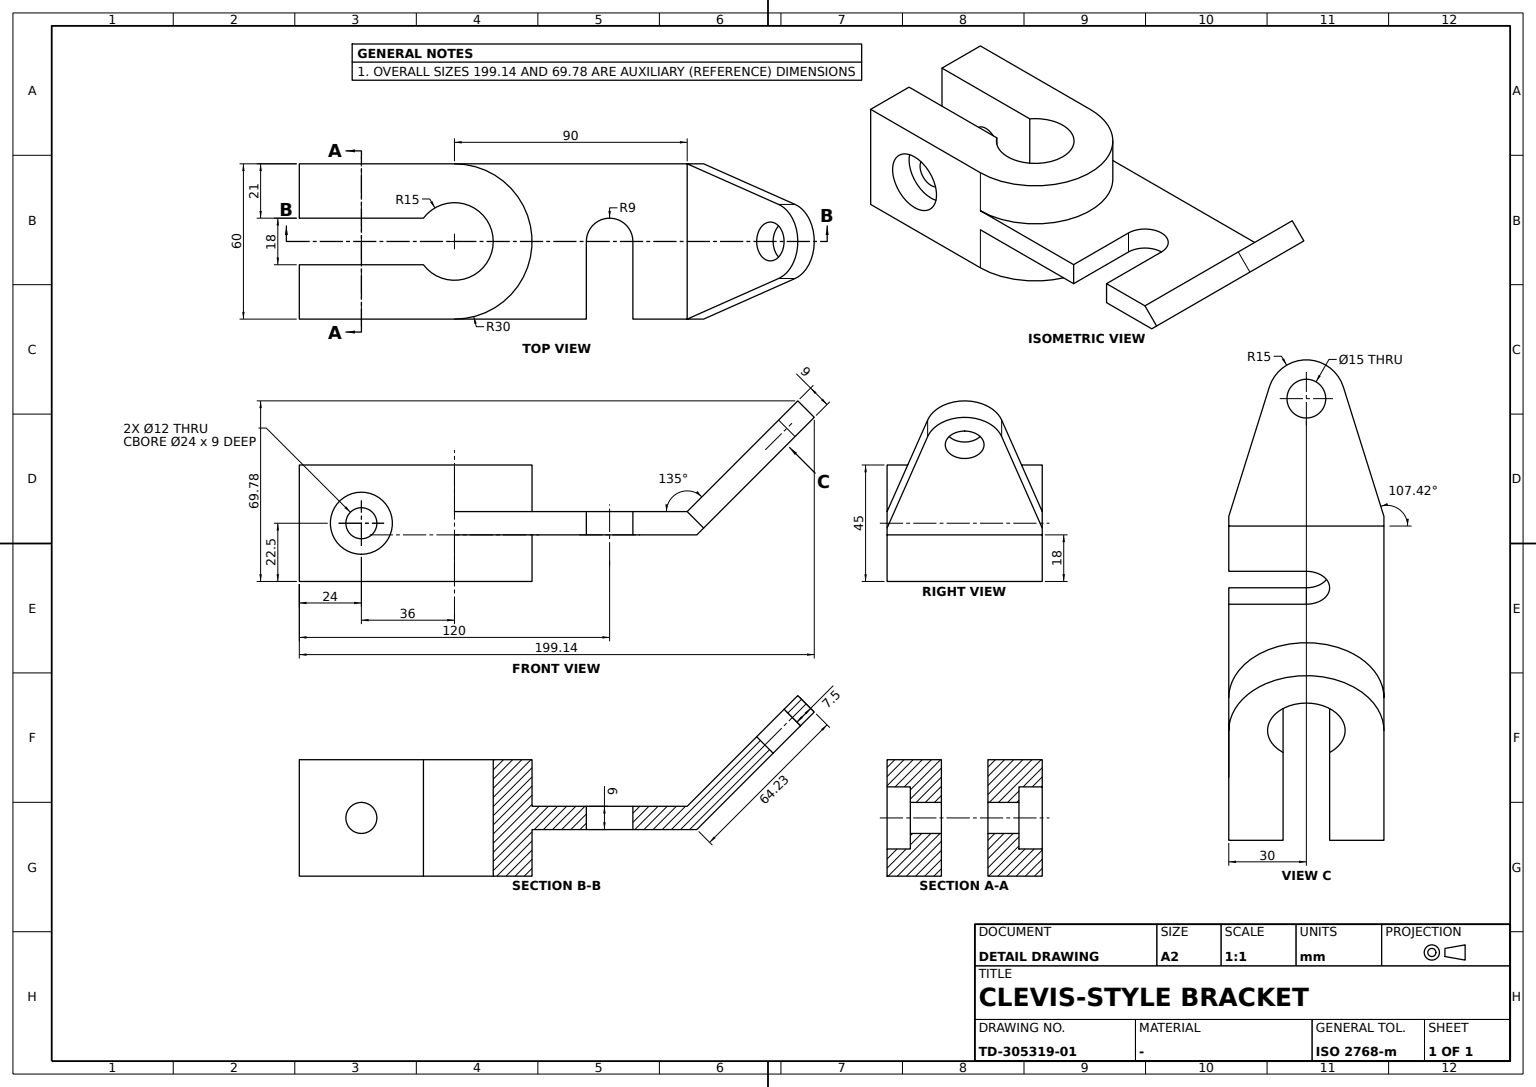
ISO-10303-21;
HEADER;
FILE_DESCRIPTION((''),'2;1');
FILE_NAME('','',(''),(''),'','','');
FILE_SCHEMA(('AUTOMOTIVE_DESIGN'));
ENDSEC;
DATA;
#1=APPLICATION_CONTEXT('');
#2=PRODUCT_CONTEXT('',#1,'mechanical');
#3=PRODUCT('','','',(#2));
#4=PRODUCT_DEFINITION_FORMATION('','',#3);
#5=PRODUCT_DEFINITION_CONTEXT('',#1,'design');
#6=PRODUCT_DEFINITION('','',#4,#5);
#7=PRODUCT_DEFINITION_SHAPE('','',#6);
#8=(LENGTH_UNIT()NAMED_UNIT(*)SI_UNIT(.MILLI.,.METRE.));
#9=(NAMED_UNIT(*)PLANE_ANGLE_UNIT()SI_UNIT($,.RADIAN.));
#10=(NAMED_UNIT(*)SI_UNIT($,.STERADIAN.)SOLID_ANGLE_UNIT());
#11=UNCERTAINTY_MEASURE_WITH_UNIT(LENGTH_MEASURE(0.005),#8,'distance_accuracy_value','');
#12=(GEOMETRIC_REPRESENTATION_CONTEXT(3)GLOBAL_UNCERTAINTY_ASSIGNED_CONTEXT((#11))GLOBAL_UNIT_ASSIGNED_CONTEXT((#8,#9,#10))REPRESENTATION_CONTEXT('',''));
#13=CARTESIAN_POINT('',(21.,-36.,6.));
#14=VERTEX_POINT('',#13);
#15=CARTESIAN_POINT('',(21.,-36.,0.));
#16=DIRECTION('',(-1.,0.,0.));
#17=DIRECTION('',(0.,0.,1.));
#18=AXIS2_PLACEMENT_3D('',#15,#16,#17);
#19=CIRCLE('',#18,6.);
#20=EDGE_CURVE('',#14,#14,#19,.T.);
#21=ORIENTED_EDGE('',*,*,#20,.T.);
#22=EDGE_LOOP('',(#21));
#23=FACE_BOUND('',#22,.T.);
#24=CARTESIAN_POINT('',(21.,-36.,12.));
#25=VERTEX_POINT('',#24);
#26=CIRCLE('',#18,12.);
#27=EDGE_CURVE('',#25,#25,#26,.T.);
#28=ORIENTED_EDGE('',*,*,#27,.F.);
#29=EDGE_LOOP('',(#28));
#30=FACE_BOUND('',#29,.T.);
#31=CARTESIAN_POINT('',(21.,-30.,0.));
#32=DIRECTION('',(0.,1.,0.));
#33=AXIS2_PLACEMENT_3D('',#31,#16,#32);
#34=PLANE('',#33);
#35=ADVANCED_FACE('',(#23,#30),#34,.F.);
#36=CARTESIAN_POINT('',(-30.,0.,22.5));
#37=VERTEX_POINT('',#36);
#38=CARTESIAN_POINT('',(-30.,-60.,22.5));
#39=VERTEX_POINT('',#38);
#40=DIRECTION('',(0.,-1.,0.));
#41=VECTOR('',#40,1000.);
#42=LINE('',#36,#41);
#43=EDGE_CURVE('',#37,#39,#42,.T.);
#44=ORIENTED_EDGE('',*,*,#43,.F.);
#45=CARTESIAN_POINT('',(-30.,0.,4.5));
#46=VERTEX_POINT('',#45);
#47=CARTESIAN_POINT('',(-30.,0.,0.));
#48=VECTOR('',#17,1000.);
#49=LINE('',#47,#48);
#50=EDGE_CURVE('',#46,#37,#49,.T.);
#51=ORIENTED_EDGE('',*,*,#50,.F.);
#52=CARTESIAN_POINT('',(-30.,90.,4.5));
#53=VERTEX_POINT('',#52);
#54=LINE('',#52,#41);
#55=EDGE_CURVE('',#53,#46,#54,.T.);
#56=ORIENTED_EDGE('',*,*,#55,.F.);
#57=CARTESIAN_POINT('',(-30.,96.363961,-1.863961));
#58=VERTEX_POINT('',#57);
#59=CARTESIAN_POINT('',(-30.,47.25,47.25));
#60=DIRECTION('',(0.,0.707106781,-0.707106781));
#61=VECTOR('',#60,1000.);
#62=LINE('',#59,#61);
#63=EDGE_CURVE('',#53,#58,#62,.T.);
#64=ORIENTED_EDGE('',*,*,#63,.T.);
#65=CARTESIAN_POINT('',(-30.,93.727922,-4.5));
#66=VERTEX_POINT('',#65);
#67=DIRECTION('',(0.,0.707106781,0.707106781));
#68=VECTOR('',#67,1000.);
#69=LINE('',#65,#68);
#70=EDGE_CURVE('',#66,#58,#69,.T.);
#71=ORIENTED_EDGE('',*,*,#70,.F.);
#72=CARTESIAN_POINT('',(-30.,0.,-4.5));
#73=VERTEX_POINT('',#72);
#74=VECTOR('',#32,1000.);
#75=LINE('',#72,#74);
#76=EDGE_CURVE('',#73,#66,#75,.T.);
#77=ORIENTED_EDGE('',*,*,#76,.F.);
#78=CARTESIAN_POINT('',(-30.,0.,-22.5));
#79=VERTEX_POINT('',#78);
#80=EDGE_CURVE('',#79,#73,#49,.T.);
#81=ORIENTED_EDGE('',*,*,#80,.F.);
#82=CARTESIAN_POINT('',(-30.,-60.,-22.5));
#83=VERTEX_POINT('',#82);
#84=LINE('',#78,#41);
#85=EDGE_CURVE('',#79,#83,#84,.T.);
#86=ORIENTED_EDGE('',*,*,#85,.T.);
#87=CARTESIAN_POINT('',(-30.,-60.,0.));
#88=LINE('',#87,#48);
#89=EDGE_CURVE('',#83,#39,#88,.T.);
#90=ORIENTED_EDGE('',*,*,#89,.T.);
#91=EDGE_LOOP('',(#44,#51,#56,#64,#71,#77,#81,#86,#90));
#92=FACE_BOUND('',#91,.T.);
#93=CARTESIAN_POINT('',(-30.,-36.,12.));
#94=VERTEX_POINT('',#93);
#95=CARTESIAN_POINT('',(-30.,-36.,0.));
#96=AXIS2_PLACEMENT_3D('',#95,#16,#17);
#97=CIRCLE('',#96,12.);
#98=EDGE_CURVE('',#94,#94,#97,.T.);
#99=ORIENTED_EDGE('',*,*,#98,.F.);
#100=EDGE_LOOP('',(#99));
#101=FACE_BOUND('',#100,.T.);
#102=AXIS2_PLACEMENT_3D('',#47,#16,#40);
#103=PLANE('',#102);
#104=ADVANCED_FACE('',(#92,#101),#103,.T.);
#105=CARTESIAN_POINT('',(0.,69.,4.5));
#106=VERTEX_POINT('',#105);
#107=CARTESIAN_POINT('',(0.,69.,-4.5));
#108=VERTEX_POINT('',#107);
#109=CARTESIAN_POINT('',(0.,69.,-9.66));
#110=LINE('',#109,#48);
#111=EDGE_CURVE('',#106,#108,#110,.F.);
#112=ORIENTED_EDGE('',*,*,#111,.F.);
#113=CARTESIAN_POINT('',(0.,51.,4.5));
#114=VERTEX_POINT('',#113);
#115=CARTESIAN_POINT('',(0.,60.,4.5));
#116=DIRECTION('',(1.,0.,0.));
#117=AXIS2_PLACEMENT_3D('',#115,#17,#116);
#118=CIRCLE('',#117,9.);
#119=EDGE_CURVE('',#106,#114,#118,.T.);
#120=ORIENTED_EDGE('',*,*,#119,.T.);
#121=CARTESIAN_POINT('',(0.,51.,-4.5));
#122=VERTEX_POINT('',#121);
#123=CARTESIAN_POINT('',(0.,51.,-9.66));
#124=LINE('',#123,#48);
#125=EDGE_CURVE('',#114,#122,#124,.F.);
#126=ORIENTED_EDGE('',*,*,#125,.T.);
#127=CARTESIAN_POINT('',(0.,60.,-4.5));
#128=DIRECTION('',(0.,0.,-1.));
#129=AXIS2_PLACEMENT_3D('',#127,#128,#16);
#130=CIRCLE('',#129,9.);
#131=EDGE_CURVE('',#122,#108,#130,.T.);
#132=ORIENTED_EDGE('',*,*,#131,.T.);
#133=EDGE_LOOP('',(#112,#120,#126,#132));
#134=FACE_BOUND('',#133,.T.);
#135=CARTESIAN_POINT('',(0.,60.,-9.66));
#136=AXIS2_PLACEMENT_3D('',#135,#17,#116);
#137=CYLINDRICAL_SURFACE('',#136,9.);
#138=ADVANCED_FACE('',(#134),#137,.F.);
#139=CARTESIAN_POINT('',(9.,-36.,-6.));
#140=VERTEX_POINT('',#139);
#141=CARTESIAN_POINT('',(9.,-36.,0.));
#142=AXIS2_PLACEMENT_3D('',#141,#116,#128);
#143=CIRCLE('',#142,6.);
#144=EDGE_CURVE('',#140,#140,#143,.T.);
#145=ORIENTED_EDGE('',*,*,#144,.F.);
#146=EDGE_LOOP('',(#145));
#147=FACE_BOUND('',#146,.T.);
#148=ORIENTED_EDGE('',*,*,#20,.F.);
#149=EDGE_LOOP('',(#148));
#150=FACE_BOUND('',#149,.T.);
#151=CARTESIAN_POINT('',(-29.9,-36.,0.));
#152=AXIS2_PLACEMENT_3D('',#151,#116,#32);
#153=CYLINDRICAL_SURFACE('',#152,6.);
#154=ADVANCED_FACE('',(#147,#150),#153,.F.);
#155=CARTESIAN_POINT('',(30.,0.,4.5));
#156=VERTEX_POINT('',#155);
#157=CARTESIAN_POINT('',(30.,0.,22.5));
#158=VERTEX_POINT('',#157);
#159=CARTESIAN_POINT('',(30.,0.,0.));
#160=LINE('',#159,#48);
#161=EDGE_CURVE('',#156,#158,#160,.T.);
#162=ORIENTED_EDGE('',*,*,#161,.F.);
#163=CARTESIAN_POINT('',(0.,0.,4.5));
#164=AXIS2_PLACEMENT_3D('',#163,#17,#116);
#165=CIRCLE('',#164,30.);
#166=EDGE_CURVE('',#156,#46,#165,.T.);
#167=ORIENTED_EDGE('',*,*,#166,.T.);
#168=ORIENTED_EDGE('',*,*,#50,.T.);
#169=CARTESIAN_POINT('',(0.,0.,22.5));
#170=AXIS2_PLACEMENT_3D('',#169,#17,#116);
#171=CIRCLE('',#170,30.);
#172=EDGE_CURVE('',#158,#37,#171,.T.);
#173=ORIENTED_EDGE('',*,*,#172,.F.);
#174=EDGE_LOOP('',(#162,#167,#168,#173));
#175=FACE_BOUND('',#174,.T.);
#176=CARTESIAN_POINT('',(0.,0.,0.));
#177=AXIS2_PLACEMENT_3D('',#176,#17,#32);
#178=CYLINDRICAL_SURFACE('',#177,30.);
#179=ADVANCED_FACE('',(#175),#178,.T.);
#180=ORIENTED_EDGE('',*,*,#144,.T.);
#181=EDGE_LOOP('',(#180));
#182=FACE_BOUND('',#181,.T.);
#183=CARTESIAN_POINT('',(9.,-12.,-22.5));
#184=VERTEX_POINT('',#183);
#185=CARTESIAN_POINT('',(9.,-60.,-22.5));
#186=VERTEX_POINT('',#185);
#187=LINE('',#183,#41);
#188=EDGE_CURVE('',#184,#186,#187,.T.);
#189=ORIENTED_EDGE('',*,*,#188,.T.);
#190=CARTESIAN_POINT('',(9.,-60.,22.5));
#191=VERTEX_POINT('',#190);
#192=CARTESIAN_POINT('',(9.,-60.,0.));
#193=VECTOR('',#128,1000.);
#194=LINE('',#192,#193);
#195=EDGE_CURVE('',#191,#186,#194,.T.);
#196=ORIENTED_EDGE('',*,*,#195,.F.);
#197=CARTESIAN_POINT('',(9.,-12.,22.5));
#198=VERTEX_POINT('',#197);
#199=LINE('',#197,#41);
#200=EDGE_CURVE('',#198,#191,#199,.T.);
#201=ORIENTED_EDGE('',*,*,#200,.F.);
#202=LINE('',#197,#48);
#203=EDGE_CURVE('',#198,#184,#202,.F.);
#204=ORIENTED_EDGE('',*,*,#203,.T.);
#205=EDGE_LOOP('',(#189,#196,#201,#204));
#206=FACE_BOUND('',#205,.T.);
#207=CARTESIAN_POINT('',(9.,-12.,0.));
#208=AXIS2_PLACEMENT_3D('',#207,#116,#40);
#209=PLANE('',#208);
#210=ADVANCED_FACE('',(#182,#206),#209,.F.);
#211=CARTESIAN_POINT('',(30.,93.727922,-4.5));
#212=VERTEX_POINT('',#211);
#213=CARTESIAN_POINT('',(30.,96.363961,-1.863961));
#214=VERTEX_POINT('',#213);
#215=CARTESIAN_POINT('',(30.,19.113961,-79.113961));
#216=LINE('',#215,#68);
#217=EDGE_CURVE('',#212,#214,#216,.T.);
#218=ORIENTED_EDGE('',*,*,#217,.T.);
#219=CARTESIAN_POINT('',(30.,90.,4.5));
#220=VERTEX_POINT('',#219);
#221=LINE('',#219,#61);
#222=EDGE_CURVE('',#220,#214,#221,.T.);
#223=ORIENTED_EDGE('',*,*,#222,.F.);
#224=CARTESIAN_POINT('',(30.,69.,4.5));
#225=VERTEX_POINT('',#224);
#226=CARTESIAN_POINT('',(30.,-60.,4.5));
#227=LINE('',#226,#41);
#228=EDGE_CURVE('',#220,#225,#227,.T.);
#229=ORIENTED_EDGE('',*,*,#228,.T.);
#230=CARTESIAN_POINT('',(30.,69.,-4.5));
#231=VERTEX_POINT('',#230);
#232=LINE('',#224,#193);
#233=EDGE_CURVE('',#225,#231,#232,.T.);
#234=ORIENTED_EDGE('',*,*,#233,.T.);
#235=CARTESIAN_POINT('',(30.,-60.,-4.5));
#236=LINE('',#235,#74);
#237=EDGE_CURVE('',#231,#212,#236,.T.);
#238=ORIENTED_EDGE('',*,*,#237,.T.);
#239=EDGE_LOOP('',(#218,#223,#229,#234,#238));
#240=FACE_BOUND('',#239,.T.);
#241=CARTESIAN_POINT('',(30.,-60.,0.));
#242=AXIS2_PLACEMENT_3D('',#241,#116,#32);
#243=PLANE('',#242);
#244=ADVANCED_FACE('',(#240),#243,.T.);
#245=CARTESIAN_POINT('',(30.,51.,4.5));
#246=VERTEX_POINT('',#245);
#247=CARTESIAN_POINT('',(30.,51.,-4.5));
#248=VERTEX_POINT('',#247);
#249=CARTESIAN_POINT('',(30.,51.,0.));
#250=LINE('',#249,#193);
#251=EDGE_CURVE('',#246,#248,#250,.T.);
#252=ORIENTED_EDGE('',*,*,#251,.T.);
#253=VECTOR('',#16,1000.);
#254=LINE('',#121,#253);
#255=EDGE_CURVE('',#248,#122,#254,.T.);
#256=ORIENTED_EDGE('',*,*,#255,.T.);
#257=ORIENTED_EDGE('',*,*,#125,.F.);
#258=LINE('',#245,#253);
#259=EDGE_CURVE('',#246,#114,#258,.T.);
#260=ORIENTED_EDGE('',*,*,#259,.F.);
#261=EDGE_LOOP('',(#252,#256,#257,#260));
#262=FACE_BOUND('',#261,.T.);
#263=AXIS2_PLACEMENT_3D('',#245,#40,#16);
#264=PLANE('',#263);
#265=ADVANCED_FACE('',(#262),#264,.F.);
#266=CARTESIAN_POINT('',(-9.,-60.,22.5));
#267=VERTEX_POINT('',#266);
#268=CARTESIAN_POINT('',(-9.,-60.,-22.5));
#269=VERTEX_POINT('',#268);
#270=CARTESIAN_POINT('',(-9.,-60.,0.));
#271=LINE('',#270,#193);
#272=EDGE_CURVE('',#267,#269,#271,.T.);
#273=ORIENTED_EDGE('',*,*,#272,.T.);
#274=CARTESIAN_POINT('',(-9.,-12.,-22.5));
#275=VERTEX_POINT('',#274);
#276=LINE('',#268,#74);
#277=EDGE_CURVE('',#269,#275,#276,.T.);
#278=ORIENTED_EDGE('',*,*,#277,.T.);
#279=CARTESIAN_POINT('',(-9.,-12.,22.5));
#280=VERTEX_POINT('',#279);
#281=LINE('',#279,#48);
#282=EDGE_CURVE('',#280,#275,#281,.F.);
#283=ORIENTED_EDGE('',*,*,#282,.F.);
#284=LINE('',#266,#74);
#285=EDGE_CURVE('',#267,#280,#284,.T.);
#286=ORIENTED_EDGE('',*,*,#285,.F.);
#287=EDGE_LOOP('',(#273,#278,#283,#286));
#288=FACE_BOUND('',#287,.T.);
#289=CARTESIAN_POINT('',(-9.,-36.,6.));
#290=VERTEX_POINT('',#289);
#291=CARTESIAN_POINT('',(-9.,-36.,0.));
#292=AXIS2_PLACEMENT_3D('',#291,#16,#17);
#293=CIRCLE('',#292,6.);
#294=EDGE_CURVE('',#290,#290,#293,.T.);
#295=ORIENTED_EDGE('',*,*,#294,.T.);
#296=EDGE_LOOP('',(#295));
#297=FACE_BOUND('',#296,.T.);
#298=AXIS2_PLACEMENT_3D('',#270,#16,#32);
#299=PLANE('',#298);
#300=ADVANCED_FACE('',(#288,#297),#299,.F.);
#301=CARTESIAN_POINT('',(30.,-60.,22.5));
#302=VERTEX_POINT('',#301);
#303=LINE('',#157,#74);
#304=EDGE_CURVE('',#302,#158,#303,.T.);
#305=ORIENTED_EDGE('',*,*,#304,.T.);
#306=ORIENTED_EDGE('',*,*,#172,.T.);
#307=ORIENTED_EDGE('',*,*,#43,.T.);
#308=CARTESIAN_POINT('',(0.,-60.,22.5));
#309=LINE('',#308,#253);
#310=EDGE_CURVE('',#267,#39,#309,.T.);
#311=ORIENTED_EDGE('',*,*,#310,.F.);
#312=ORIENTED_EDGE('',*,*,#285,.T.);
#313=CIRCLE('',#170,15.);
#314=EDGE_CURVE('',#198,#280,#313,.T.);
#315=ORIENTED_EDGE('',*,*,#314,.F.);
#316=ORIENTED_EDGE('',*,*,#200,.T.);
#317=EDGE_CURVE('',#302,#191,#309,.T.);
#318=ORIENTED_EDGE('',*,*,#317,.F.);
#319=EDGE_LOOP('',(#305,#306,#307,#311,#312,#315,#316,#318));
#320=FACE_BOUND('',#319,.T.);
#321=AXIS2_PLACEMENT_3D('',#169,#17,#32);
#322=PLANE('',#321);
#323=ADVANCED_FACE('',(#320),#322,.T.);
#324=CARTESIAN_POINT('',(-21.,-36.,-12.));
#325=VERTEX_POINT('',#324);
#326=CARTESIAN_POINT('',(-21.,-36.,0.));
#327=AXIS2_PLACEMENT_3D('',#326,#116,#128);
#328=CIRCLE('',#327,12.);
#329=EDGE_CURVE('',#325,#325,#328,.T.);
#330=ORIENTED_EDGE('',*,*,#329,.F.);
#331=EDGE_LOOP('',(#330));
#332=FACE_BOUND('',#331,.T.);
#333=CARTESIAN_POINT('',(-21.,-36.,-6.));
#334=VERTEX_POINT('',#333);
#335=CIRCLE('',#327,6.);
#336=EDGE_CURVE('',#334,#334,#335,.T.);
#337=ORIENTED_EDGE('',*,*,#336,.T.);
#338=EDGE_LOOP('',(#337));
#339=FACE_BOUND('',#338,.T.);
#340=CARTESIAN_POINT('',(-21.,-30.,0.));
#341=AXIS2_PLACEMENT_3D('',#340,#116,#32);
#342=PLANE('',#341);
#343=ADVANCED_FACE('',(#332,#339),#342,.F.);
#344=ORIENTED_EDGE('',*,*,#294,.F.);
#345=EDGE_LOOP('',(#344));
#346=FACE_BOUND('',#345,.T.);
#347=ORIENTED_EDGE('',*,*,#336,.F.);
#348=EDGE_LOOP('',(#347));
#349=FACE_BOUND('',#348,.T.);
#350=ADVANCED_FACE('',(#346,#349),#153,.F.);
#351=CARTESIAN_POINT('',(30.,0.,-22.5));
#352=VERTEX_POINT('',#351);
#353=CARTESIAN_POINT('',(30.,0.,-4.5));
#354=VERTEX_POINT('',#353);
#355=EDGE_CURVE('',#352,#354,#160,.T.);
#356=ORIENTED_EDGE('',*,*,#355,.F.);
#357=CARTESIAN_POINT('',(0.,0.,-22.5));
#358=AXIS2_PLACEMENT_3D('',#357,#17,#116);
#359=CIRCLE('',#358,30.);
#360=EDGE_CURVE('',#352,#79,#359,.T.);
#361=ORIENTED_EDGE('',*,*,#360,.T.);
#362=ORIENTED_EDGE('',*,*,#80,.T.);
#363=CARTESIAN_POINT('',(0.,0.,-4.5));
#364=AXIS2_PLACEMENT_3D('',#363,#128,#16);
#365=CIRCLE('',#364,30.);
#366=EDGE_CURVE('',#73,#354,#365,.T.);
#367=ORIENTED_EDGE('',*,*,#366,.T.);
#368=EDGE_LOOP('',(#356,#361,#362,#367));
#369=FACE_BOUND('',#368,.T.);
#370=ADVANCED_FACE('',(#369),#178,.T.);
#371=LINE('',#107,#253);
#372=EDGE_CURVE('',#231,#108,#371,.T.);
#373=ORIENTED_EDGE('',*,*,#372,.F.);
#374=ORIENTED_EDGE('',*,*,#233,.F.);
#375=VECTOR('',#116,1000.);
#376=LINE('',#105,#375);
#377=EDGE_CURVE('',#106,#225,#376,.T.);
#378=ORIENTED_EDGE('',*,*,#377,.F.);
#379=ORIENTED_EDGE('',*,*,#111,.T.);
#380=EDGE_LOOP('',(#373,#374,#378,#379));
#381=FACE_BOUND('',#380,.T.);
#382=AXIS2_PLACEMENT_3D('',#105,#32,#116);
#383=PLANE('',#382);
#384=ADVANCED_FACE('',(#381),#383,.F.);
#385=CARTESIAN_POINT('',(-14.311818,125.349193,39.849193));
#386=VERTEX_POINT('',#385);
#387=CARTESIAN_POINT('',(-14.311818,131.713154,33.485232));
#388=VERTEX_POINT('',#387);
#389=CARTESIAN_POINT('',(-14.311818,133.304145,31.894242));
#390=DIRECTION('',(0.,-0.707106781,0.707106781));
#391=VECTOR('',#390,1000.);
#392=LINE('',#389,#391);
#393=EDGE_CURVE('',#386,#388,#392,.F.);
#394=ORIENTED_EDGE('',*,*,#393,.F.);
#395=CARTESIAN_POINT('',(14.311818,125.349193,39.849193));
#396=VERTEX_POINT('',#395);
#397=CARTESIAN_POINT('',(0.,122.173359,36.673359));
#398=DIRECTION('',(0.,-0.707106781,-0.707106781));
#399=AXIS2_PLACEMENT_3D('',#397,#390,#398);
#400=CIRCLE('',#399,15.);
#401=EDGE_CURVE('',#396,#386,#400,.T.);
#402=ORIENTED_EDGE('',*,*,#401,.F.);
#403=CARTESIAN_POINT('',(14.311818,131.713154,33.485232));
#404=VERTEX_POINT('',#403);
#405=CARTESIAN_POINT('',(14.311818,133.304145,31.894242));
#406=LINE('',#405,#391);
#407=EDGE_CURVE('',#396,#404,#406,.F.);
#408=ORIENTED_EDGE('',*,*,#407,.T.);
#409=CARTESIAN_POINT('',(0.,128.53732,30.309398));
#410=AXIS2_PLACEMENT_3D('',#409,#60,#67);
#411=CIRCLE('',#410,15.);
#412=EDGE_CURVE('',#388,#404,#411,.T.);
#413=ORIENTED_EDGE('',*,*,#412,.F.);
#414=EDGE_LOOP('',(#394,#402,#408,#413));
#415=FACE_BOUND('',#414,.T.);
#416=CARTESIAN_POINT('',(0.,130.12831,28.718407));
#417=AXIS2_PLACEMENT_3D('',#416,#390,#116);
#418=CYLINDRICAL_SURFACE('',#417,15.);
#419=ADVANCED_FACE('',(#415),#418,.T.);
#420=ORIENTED_EDGE('',*,*,#27,.T.);
#421=EDGE_LOOP('',(#420));
#422=FACE_BOUND('',#421,.T.);
#423=CARTESIAN_POINT('',(30.,-36.,-12.));
#424=VERTEX_POINT('',#423);
#425=CARTESIAN_POINT('',(30.,-36.,0.));
#426=AXIS2_PLACEMENT_3D('',#425,#116,#128);
#427=CIRCLE('',#426,12.);
#428=EDGE_CURVE('',#424,#424,#427,.T.);
#429=ORIENTED_EDGE('',*,*,#428,.T.);
#430=EDGE_LOOP('',(#429));
#431=FACE_BOUND('',#430,.T.);
#432=CARTESIAN_POINT('',(29.9,-36.,0.));
#433=AXIS2_PLACEMENT_3D('',#432,#16,#32);
#434=CYLINDRICAL_SURFACE('',#433,12.);
#435=ADVANCED_FACE('',(#422,#431),#434,.F.);
#436=ORIENTED_EDGE('',*,*,#407,.F.);
#437=DIRECTION('',(0.299420588,-0.674665588,-0.674665588));
#438=VECTOR('',#437,1000.);
#439=LINE('',#395,#438);
#440=EDGE_CURVE('',#396,#220,#439,.T.);
#441=ORIENTED_EDGE('',*,*,#440,.T.);
#442=ORIENTED_EDGE('',*,*,#222,.T.);
#443=DIRECTION('',(-0.299420588,0.674665588,0.674665588));
#444=VECTOR('',#443,1000.);
#445=LINE('',#403,#444);
#446=EDGE_CURVE('',#214,#404,#445,.T.);
#447=ORIENTED_EDGE('',*,*,#446,.T.);
#448=EDGE_LOOP('',(#436,#441,#442,#447));
#449=FACE_BOUND('',#448,.T.);
#450=DIRECTION('',(0.954121225,0.211722328,0.211722328));
#451=AXIS2_PLACEMENT_3D('',#395,#450,#437);
#452=PLANE('',#451);
#453=ADVANCED_FACE('',(#449),#452,.T.);
#454=ORIENTED_EDGE('',*,*,#188,.F.);
#455=CIRCLE('',#358,15.);
#456=EDGE_CURVE('',#184,#275,#455,.T.);
#457=ORIENTED_EDGE('',*,*,#456,.T.);
#458=ORIENTED_EDGE('',*,*,#277,.F.);
#459=CARTESIAN_POINT('',(0.,-60.,-22.5));
#460=LINE('',#459,#253);
#461=EDGE_CURVE('',#269,#83,#460,.T.);
#462=ORIENTED_EDGE('',*,*,#461,.T.);
#463=ORIENTED_EDGE('',*,*,#85,.F.);
#464=ORIENTED_EDGE('',*,*,#360,.F.);
#465=CARTESIAN_POINT('',(30.,-60.,-22.5));
#466=VERTEX_POINT('',#465);
#467=LINE('',#351,#74);
#468=EDGE_CURVE('',#466,#352,#467,.T.);
#469=ORIENTED_EDGE('',*,*,#468,.F.);
#470=EDGE_CURVE('',#466,#186,#460,.T.);
#471=ORIENTED_EDGE('',*,*,#470,.T.);
#472=EDGE_LOOP('',(#454,#457,#458,#462,#463,#464,#469,#471));
#473=FACE_BOUND('',#472,.T.);
#474=AXIS2_PLACEMENT_3D('',#357,#17,#32);
#475=PLANE('',#474);
#476=ADVANCED_FACE('',(#473),#475,.F.);
#477=CARTESIAN_POINT('',(0.,133.84062,35.612698));
#478=VERTEX_POINT('',#477);
#479=CIRCLE('',#410,7.5);
#480=EDGE_CURVE('',#478,#478,#479,.T.);
#481=ORIENTED_EDGE('',*,*,#480,.F.);
#482=EDGE_LOOP('',(#481));
#483=FACE_BOUND('',#482,.T.);
#484=ORIENTED_EDGE('',*,*,#446,.F.);
#485=ORIENTED_EDGE('',*,*,#217,.F.);
#486=CARTESIAN_POINT('',(0.,93.727922,-4.5));
#487=LINE('',#486,#375);
#488=EDGE_CURVE('',#66,#212,#487,.T.);
#489=ORIENTED_EDGE('',*,*,#488,.F.);
#490=ORIENTED_EDGE('',*,*,#70,.T.);
#491=CARTESIAN_POINT('',(-28.375425,100.024513,1.796591));
#492=DIRECTION('',(0.299420588,0.674665588,0.674665588));
#493=VECTOR('',#492,1000.);
#494=LINE('',#491,#493);
#495=EDGE_CURVE('',#58,#388,#494,.T.);
#496=ORIENTED_EDGE('',*,*,#495,.T.);
#497=ORIENTED_EDGE('',*,*,#412,.T.);
#498=EDGE_LOOP('',(#484,#485,#489,#490,#496,#497));
#499=FACE_BOUND('',#498,.T.);
#500=AXIS2_PLACEMENT_3D('',#486,#60,#67);
#501=PLANE('',#500);
#502=ADVANCED_FACE('',(#483,#499),#501,.T.);
#503=ORIENTED_EDGE('',*,*,#251,.F.);
#504=EDGE_CURVE('',#246,#156,#227,.T.);
#505=ORIENTED_EDGE('',*,*,#504,.T.);
#506=ORIENTED_EDGE('',*,*,#161,.T.);
#507=ORIENTED_EDGE('',*,*,#304,.F.);
#508=LINE('',#241,#48);
#509=EDGE_CURVE('',#466,#302,#508,.T.);
#510=ORIENTED_EDGE('',*,*,#509,.F.);
#511=ORIENTED_EDGE('',*,*,#468,.T.);
#512=ORIENTED_EDGE('',*,*,#355,.T.);
#513=EDGE_CURVE('',#354,#248,#236,.T.);
#514=ORIENTED_EDGE('',*,*,#513,.T.);
#515=EDGE_LOOP('',(#503,#505,#506,#507,#510,#511,#512,#514));
#516=FACE_BOUND('',#515,.T.);
#517=ORIENTED_EDGE('',*,*,#428,.F.);
#518=EDGE_LOOP('',(#517));
#519=FACE_BOUND('',#518,.T.);
#520=ADVANCED_FACE('',(#516,#519),#243,.T.);
#521=ORIENTED_EDGE('',*,*,#259,.T.);
#522=ORIENTED_EDGE('',*,*,#119,.F.);
#523=ORIENTED_EDGE('',*,*,#377,.T.);
#524=ORIENTED_EDGE('',*,*,#228,.F.);
#525=CARTESIAN_POINT('',(0.,90.,4.5));
#526=LINE('',#525,#375);
#527=EDGE_CURVE('',#53,#220,#526,.T.);
#528=ORIENTED_EDGE('',*,*,#527,.F.);
#529=ORIENTED_EDGE('',*,*,#55,.T.);
#530=ORIENTED_EDGE('',*,*,#166,.F.);
#531=ORIENTED_EDGE('',*,*,#504,.F.);
#532=EDGE_LOOP('',(#521,#522,#523,#524,#528,#529,#530,#531));
#533=FACE_BOUND('',#532,.T.);
#534=AXIS2_PLACEMENT_3D('',#525,#17,#40);
#535=PLANE('',#534);
#536=ADVANCED_FACE('',(#533),#535,.T.);
#537=ORIENTED_EDGE('',*,*,#456,.F.);
#538=ORIENTED_EDGE('',*,*,#203,.F.);
#539=ORIENTED_EDGE('',*,*,#314,.T.);
#540=ORIENTED_EDGE('',*,*,#282,.T.);
#541=EDGE_LOOP('',(#537,#538,#539,#540));
#542=FACE_BOUND('',#541,.T.);
#543=AXIS2_PLACEMENT_3D('',#176,#17,#116);
#544=CYLINDRICAL_SURFACE('',#543,15.);
#545=ADVANCED_FACE('',(#542),#544,.F.);
#546=LINE('',#52,#493);
#547=EDGE_CURVE('',#53,#386,#546,.T.);
#548=ORIENTED_EDGE('',*,*,#547,.T.);
#549=ORIENTED_EDGE('',*,*,#393,.T.);
#550=ORIENTED_EDGE('',*,*,#495,.F.);
#551=ORIENTED_EDGE('',*,*,#63,.F.);
#552=EDGE_LOOP('',(#548,#549,#550,#551));
#553=FACE_BOUND('',#552,.T.);
#554=DIRECTION('',(-0.954121225,0.211722328,0.211722328));
#555=AXIS2_PLACEMENT_3D('',#52,#554,#492);
#556=PLANE('',#555);
#557=ADVANCED_FACE('',(#553),#556,.T.);
#558=ORIENTED_EDGE('',*,*,#461,.F.);
#559=ORIENTED_EDGE('',*,*,#272,.F.);
#560=ORIENTED_EDGE('',*,*,#310,.T.);
#561=ORIENTED_EDGE('',*,*,#89,.F.);
#562=EDGE_LOOP('',(#558,#559,#560,#561));
#563=FACE_BOUND('',#562,.T.);
#564=AXIS2_PLACEMENT_3D('',#241,#32,#16);
#565=PLANE('',#564);
#566=ADVANCED_FACE('',(#563),#565,.F.);
#567=ORIENTED_EDGE('',*,*,#372,.T.);
#568=ORIENTED_EDGE('',*,*,#131,.F.);
#569=ORIENTED_EDGE('',*,*,#255,.F.);
#570=ORIENTED_EDGE('',*,*,#513,.F.);
#571=ORIENTED_EDGE('',*,*,#366,.F.);
#572=ORIENTED_EDGE('',*,*,#76,.T.);
#573=ORIENTED_EDGE('',*,*,#488,.T.);
#574=ORIENTED_EDGE('',*,*,#237,.F.);
#575=EDGE_LOOP('',(#567,#568,#569,#570,#571,#572,#573,#574));
#576=FACE_BOUND('',#575,.T.);
#577=AXIS2_PLACEMENT_3D('',#363,#128,#32);
#578=PLANE('',#577);
#579=ADVANCED_FACE('',(#576),#578,.T.);
#580=CARTESIAN_POINT('',(0.,116.870058,31.370058));
#581=VERTEX_POINT('',#580);
#582=CIRCLE('',#399,7.5);
#583=EDGE_CURVE('',#581,#581,#582,.T.);
#584=ORIENTED_EDGE('',*,*,#583,.T.);
#585=EDGE_LOOP('',(#584));
#586=FACE_BOUND('',#585,.T.);
#587=ORIENTED_EDGE('',*,*,#480,.T.);
#588=EDGE_LOOP('',(#587));
#589=FACE_BOUND('',#588,.T.);
#590=CARTESIAN_POINT('',(0.,147.026193,11.820524));
#591=AXIS2_PLACEMENT_3D('',#590,#390,#116);
#592=CYLINDRICAL_SURFACE('',#591,7.5);
#593=ADVANCED_FACE('',(#586,#589),#592,.F.);
#594=ORIENTED_EDGE('',*,*,#98,.T.);
#595=EDGE_LOOP('',(#594));
#596=FACE_BOUND('',#595,.T.);
#597=ORIENTED_EDGE('',*,*,#329,.T.);
#598=EDGE_LOOP('',(#597));
#599=FACE_BOUND('',#598,.T.);
#600=ADVANCED_FACE('',(#596,#599),#434,.F.);
#601=ORIENTED_EDGE('',*,*,#583,.F.);
#602=EDGE_LOOP('',(#601));
#603=FACE_BOUND('',#602,.T.);
#604=ORIENTED_EDGE('',*,*,#527,.T.);
#605=ORIENTED_EDGE('',*,*,#440,.F.);
#606=ORIENTED_EDGE('',*,*,#401,.T.);
#607=ORIENTED_EDGE('',*,*,#547,.F.);
#608=EDGE_LOOP('',(#604,#605,#606,#607));
#609=FACE_BOUND('',#608,.T.);
#610=CARTESIAN_POINT('',(0.,133.84062,48.34062));
#611=AXIS2_PLACEMENT_3D('',#610,#390,#398);
#612=PLANE('',#611);
#613=ADVANCED_FACE('',(#603,#609),#612,.T.);
#614=ORIENTED_EDGE('',*,*,#509,.T.);
#615=ORIENTED_EDGE('',*,*,#317,.T.);
#616=ORIENTED_EDGE('',*,*,#195,.T.);
#617=ORIENTED_EDGE('',*,*,#470,.F.);
#618=EDGE_LOOP('',(#614,#615,#616,#617));
#619=FACE_BOUND('',#618,.T.);
#620=ADVANCED_FACE('',(#619),#565,.F.);
#621=CLOSED_SHELL('',(#35,#104,#138,#154,#179,#210,#244,#265,#300,#323,#343,#350,#370,#384,#419,#435,#453,#476,#502,#520,#536,#545,#557,#566,#579,#593,#600,#613,#620));
#622=MANIFOLD_SOLID_BREP('',#621);
#623=ADVANCED_BREP_SHAPE_REPRESENTATION('',(#622),#12);
#624=SHAPE_DEFINITION_REPRESENTATION(#7,#623);
ENDSEC;
END-ISO-10303-21;
